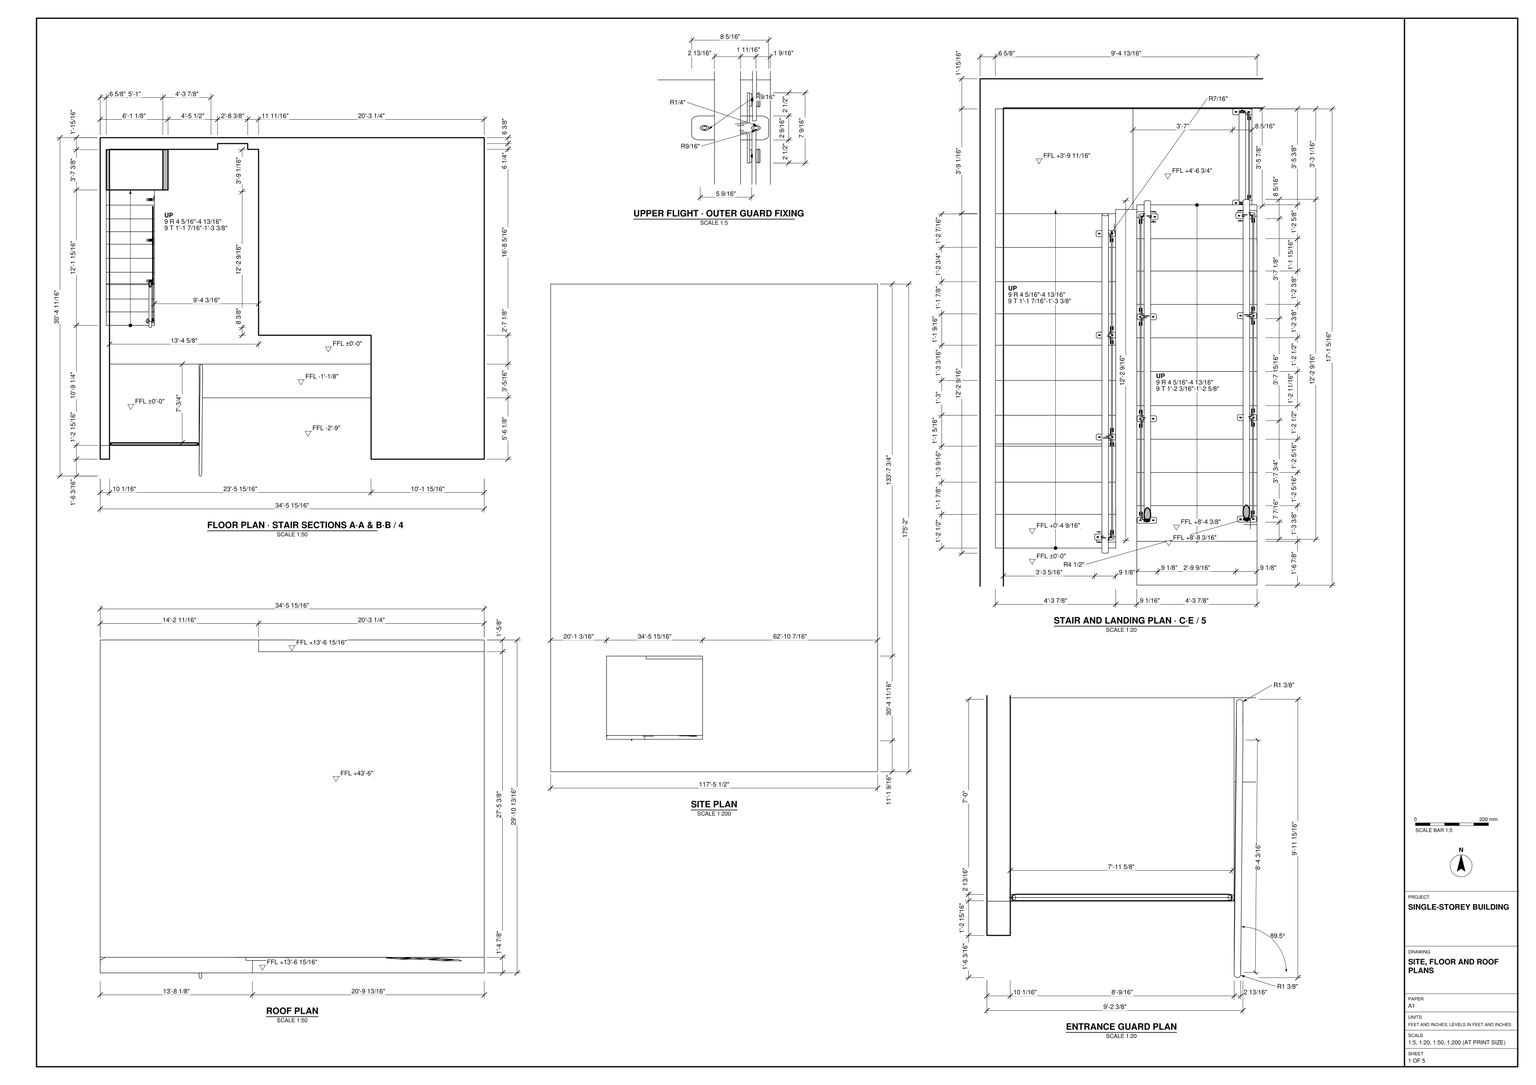
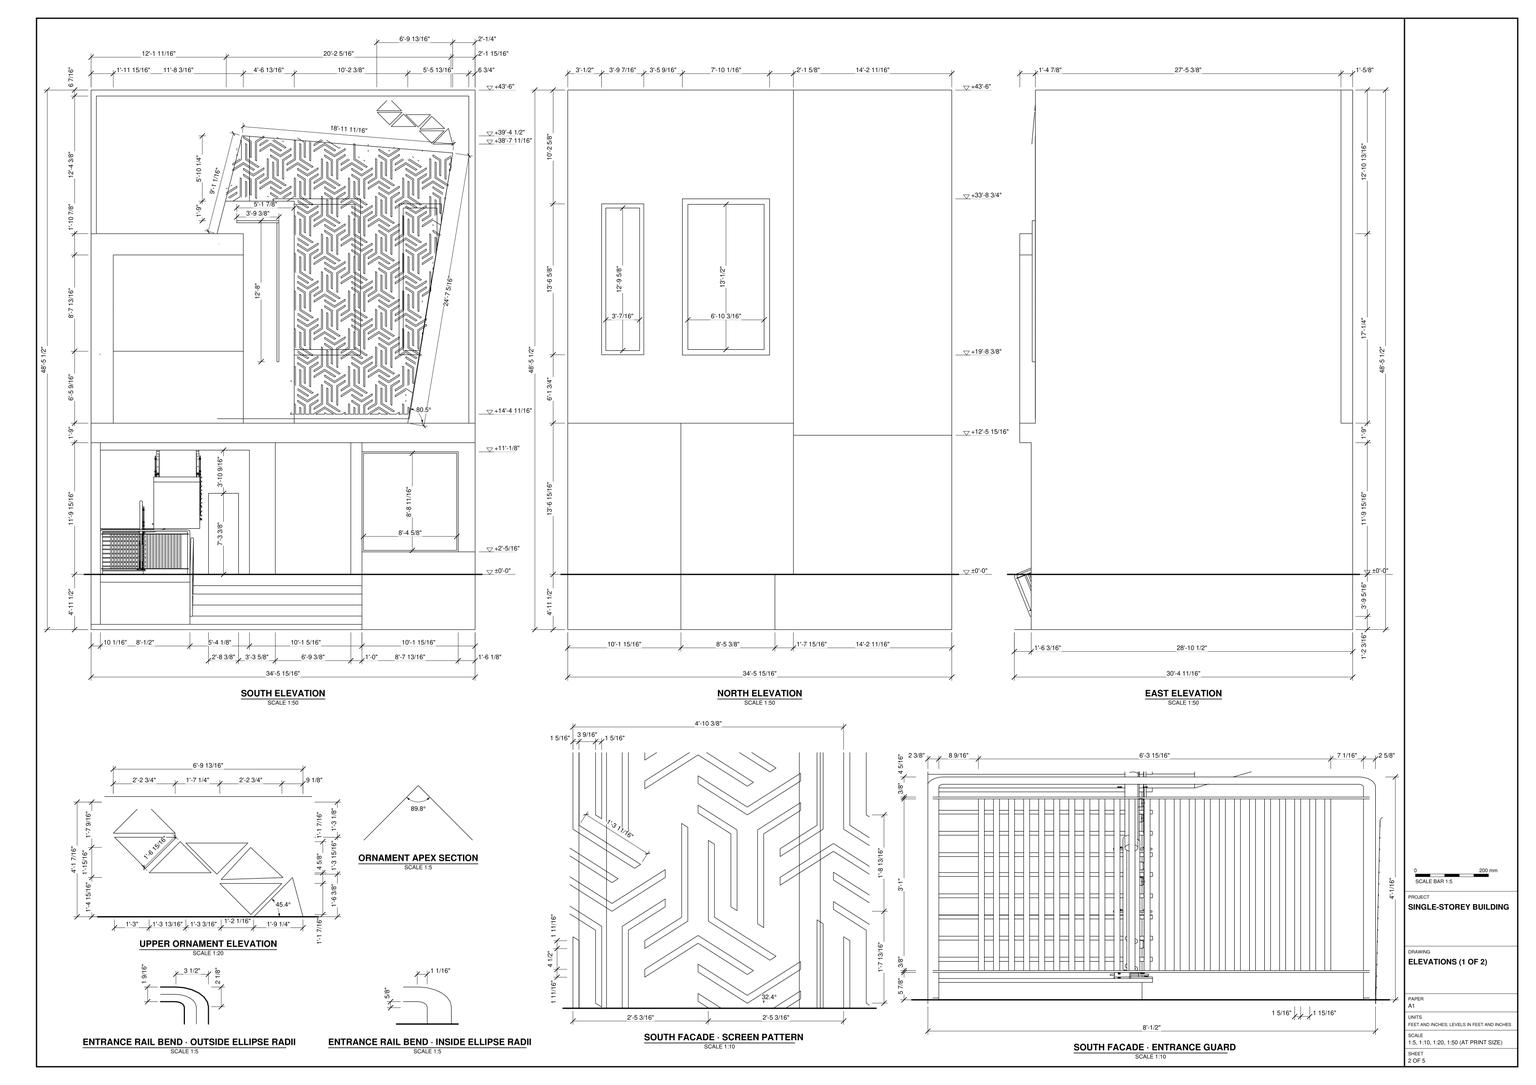
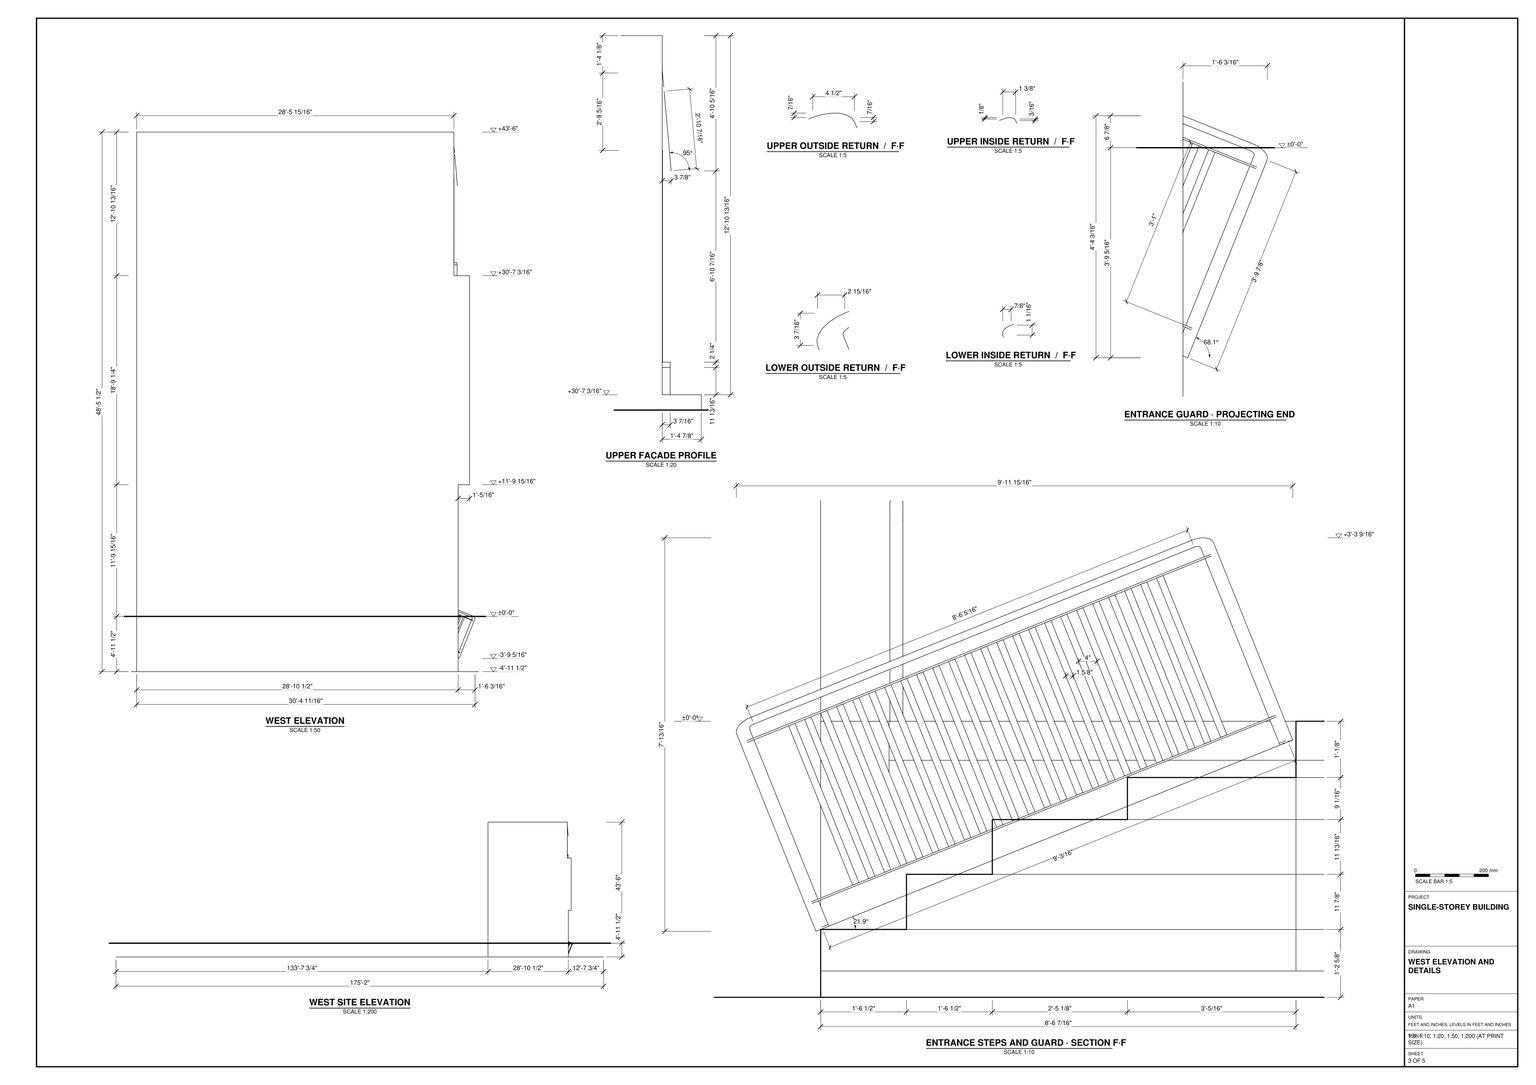
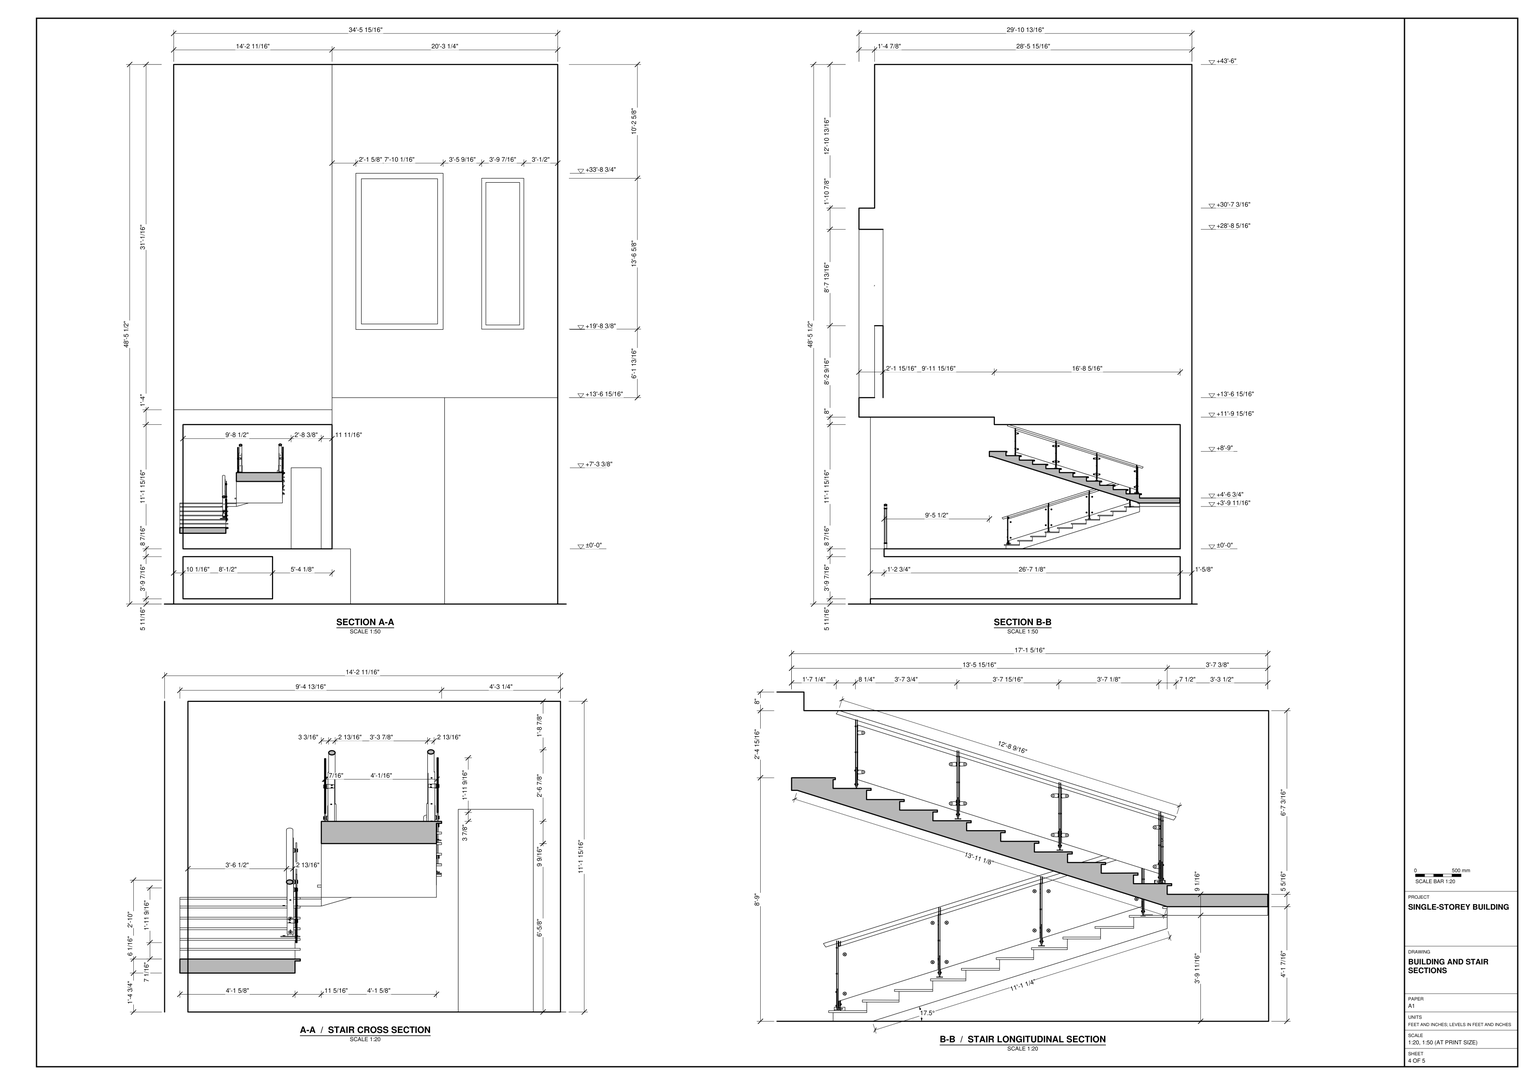
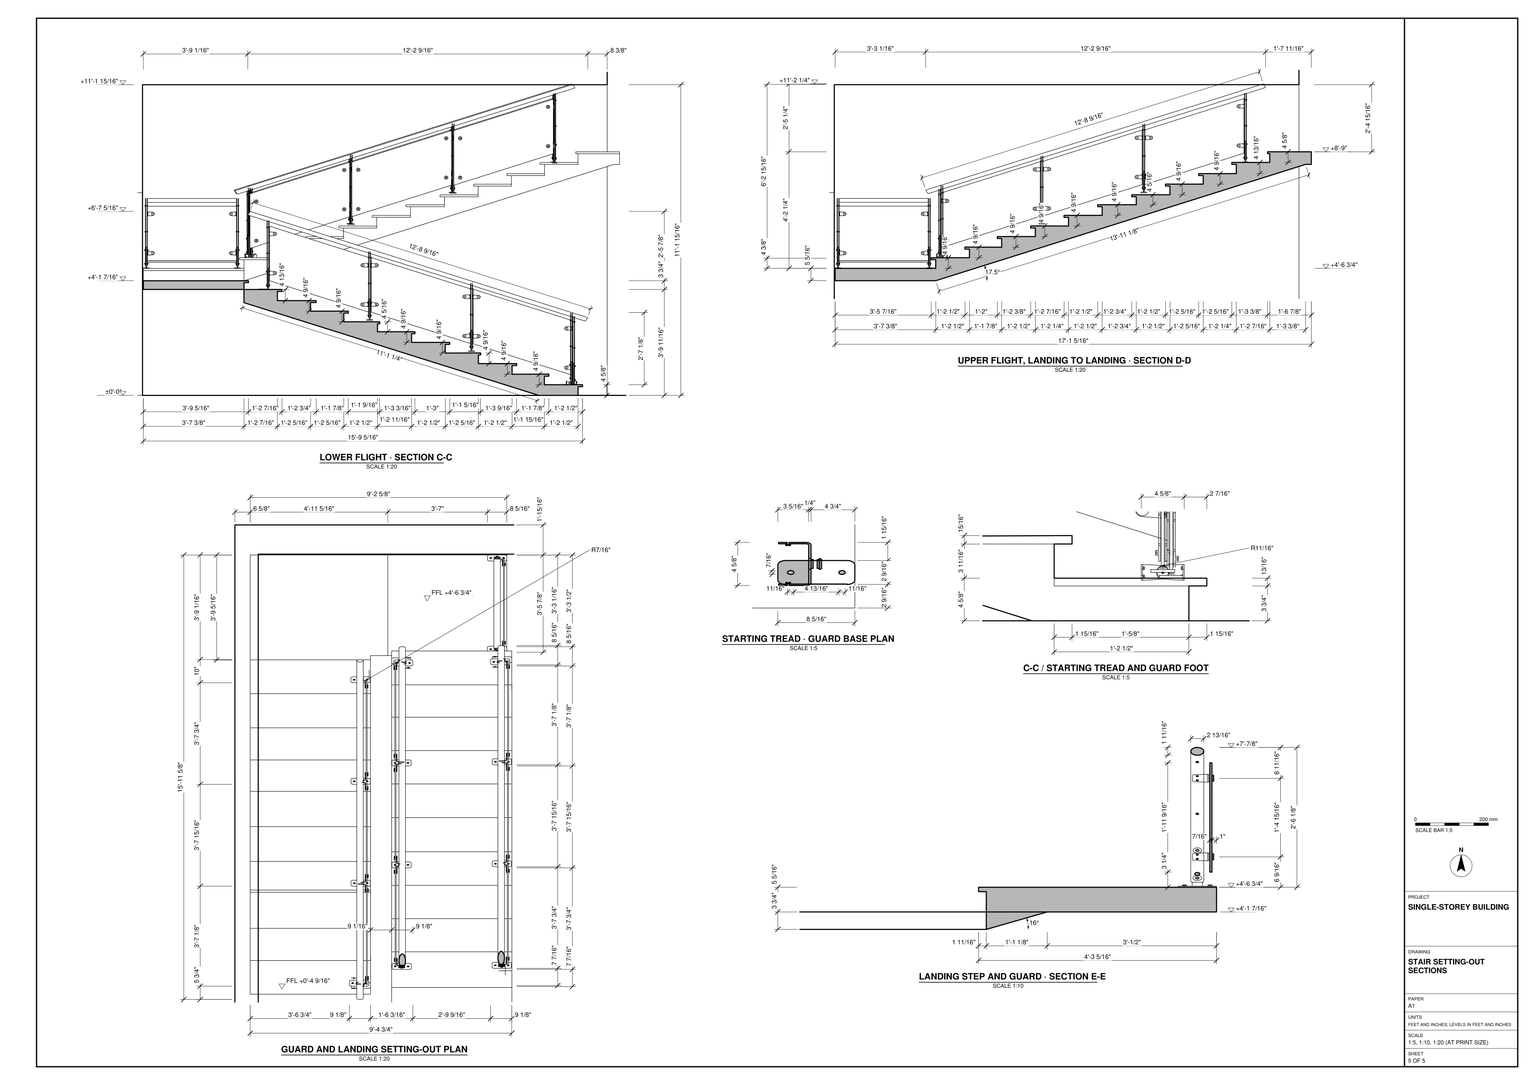
Work in feet and inches in SketchUp. Use task_files/diagram_01.pdf to model the building and its rectangular site. Including the site, the model measures 117'-5 1/2" along X, 175'-2" along Y and 48'-5 1/2" along Z. Use ±0'-0" as the ground-floor level. Position the building near the south end of the site, with more open ground to its east than to its west.

Build the walls, floor slabs and flat roof to the thicknesses and profiles shown. Use the elevations to place the framed openings and to set out the projections on the south facade. Model the sloping edges, notch and repeating angular pattern of the upper screen. Below it, form the entrance steps and landing, with the level guard across the landing and the sloping guard beside the steps. Follow the stair and landing plan for the two parallel flights; use the sections and fixing details to place the glass guards, posts and brackets along their edges.

Keep the walls, slabs and roof in separate groups or components. Group each furniture or joinery piece shown separately, and use components for repeated parts. Decor and loose items may be any suitable library components. Save one SketchUp model as output_files/single_storey_building_with_screened_facade_and_stairs.skp.

# SketchUp Ruby script. Lengths in inches.
U = 1.inch
M = Sketchup.active_model
def pt(a) = Geom::Point3d.new(a.map { |v| v * U })
def face(e, loops, mat)
  f = e.add_face(loops[0].map { |a| pt(a) })
  loops[1..].each { |l| e.add_face(l.map { |a| pt(a) }).erase! }
  f.material = f.back_material = mat if mat
  f
end
# faces: each face lists its corners as indices into pts; further lists are holes
def faces(e, pts, list, mat = nil) = list.each { |f| face(e, (f[0].is_a?(Array) ? f : [f]).map { |l| l.map { |i| pts[i] } }, mat) }
# xy, xz, yz: faces in a plane at the given z, y or x. An outline is a flat list of corners, or four numbers for a rectangle; further outlines are holes
def ring(l) = l.size == 4 ? [[l[0], l[1]], [l[2], l[1]], [l[2], l[3]], [l[0], l[3]]] : l.each_slice(2).to_a
def flat(e, list, mat, &to3) = list.each { |f| face(e, (f[0].is_a?(Array) ? f : [f]).map { |l| ring(l).map { |u, v| to3.(u, v) } }, mat) }
def xy(e, z, list, mat = nil) = flat(e, list, mat) { |x, y| [x, y, z] }
def xz(e, y, list, mat = nil) = flat(e, list, mat) { |x, z| [x, y, z] }
def yz(e, x, list, mat = nil) = flat(e, list, mat) { |y, z| [x, y, z] }
def lines(e, pts, list) = list.each { |a, b| e.add_line(pt(pts[a]), pt(pts[b])) }
# prism: a flat outline (further loops are holes) pulled along v
def prism(e, loops, v, mat = nil)
  f = face(e, loops, mat); d = Geom::Vector3d.new(v.map { |x| x * U })
  f.pushpull(f.normal.samedirection?(d) ? d.length : -d.length)
end
def box(e, o, s, mat = nil) = prism(e, [[o, [o[0] + s[0], o[1], o[2]], [o[0] + s[0], o[1] + s[1], o[2]], [o[0], o[1] + s[1], o[2]]]], [0, 0, s[2]], mat)
def at(x, y, z, deg = 0) = Geom::Transformation.translation(pt([x, y, z])) * Geom::Transformation.rotation(ORIGIN, Z_AXIS, deg.degrees)
def axes(o, x, y, z) = Geom::Transformation.new([*x, 0, *y, 0, *z, 0, *pt(o).to_a, 1])
def part(name) = M.definitions.add(name)
# library, detail: a bought-in or finely detailed component or shape, given as its bounding box
def library(name, o, s) = part(name).tap { |d| box(d.entities, o, s) }
def detail(e, o, s) = box(e.add_group.entities, o, s)
def put(e, d, t, mat = nil) = e.add_instance(d, t).tap { |i| i.material = mat if mat }
def group(e, t, mat = nil) = e.add_group.tap { |g| g.transformation = t; g.material = mat if mat }.entities
root = M.entities
M.materials.add("Niraj_Hair_Dark").color = [109, 109, 109]
M.materials.add("[0010_Snow]").color = [255, 250, 250]
M.materials.add("[Asphalt New]").color = [67, 60, 62]
M.materials.add("[Grass Dark Green]").color = [106, 157, 55]
M.materials.add("[Stone Coursed Rough]").color = [165, 160, 130]
M.materials.add("[Translucent Glass Gray]").color = [128, 128, 128]
M.materials["[Translucent Glass Gray]"].alpha = 0.5
M.materials.add("[Wood Floor Parquet]").color = [145, 89, 39]
M.materials.add("[Wood OSB]").color = [240, 195, 122]
c1 = library("Stairs\#2",[2342.14,0.12,0],[188.54,80.27,159.8125])
c2 = library("Group\#3",[1.59,0,0],[218.88,269.6875,1.18])
c3 = part("Patterned screen panel")
put(c3.entities,c2,at(3.9375,3.93,0))
c4 = part("CNC+PATTERN+DESIGN-1")
p = [[-487.64,162.15,197.43],[-460.46,162.15,303.05],[-233.53,162.15,284.47],[-280.48,162.01,-1.96],[-487.39,162.01,-1.96]]
lines(c4.entities,p,[[0,1],[1,2],[2,3],[3,4]])
put(c4.entities,c3,axes([-487.45,163.33,-1.96],[1.1232,0,0],[0,0,1.23552],[0,-1.1232,0]))
c5 = library("grille",[52.54,2.91,0],[58.66,1.57,48.03])
c6 = part("Group\#6")
xy(c6.entities,0,[[0,0,51.78,0,25.89,32]])
xy(root,0,[[241.17,151.76,655.09,498.26]])
xy(root,0,[[[0,0,1409.5,2102],[241.17,151.76,655.09,498.26]]],"[Grass Dark Green]")
xy(root,5.67,[[251.23,151.76,347.73,485.66]])
xy(root,14.625,[[347.73,151.76,533.15,170.26]])
xy(root,26.5,[[347.73,170.26,533.15,188.76]])
xy(root,38.3125,[[347.73,188.76,533.15,217.89]])
xy(root,47.375,[[347.73,217.89,533.15,254.22]])
xy(root,51.09,[[251.23,166.51,347.73,485.66]])
xy(root,59.5,[[241.17,151.76,251.23,166.51],[251.23,166.51,347.73,254.22],[251.23,254.22,533.15,254.22,533.15,285.32,411.85,285.32,411.85,485.66,400.14,485.66,400.14,491.91,367.76,491.91,367.76,485.66,251.23,485.66]])
xy(root,146.875,[[367.76,485.66,400.14,491.91]])
xy(root,193.42,[[251.23,285.32,411.85,485.66]])
xy(root,201.4375,[[241.17,139.45,251.23,151.76],[439.77,139.45,521.14,285.32],[533.15,139.45,655.09,151.76]])
xy(root,201.4375,[[251.23,139.45,439.77,285.32],[521.14,139.45,533.15,285.32]],"[Stone Coursed Rough]")
xy(root,222.4375,[[265.11,139.45,655.09,156.3],[411.85,485.66,655.09,498.26]])
xy(root,288.73,[[441.5,152.86,443.62,156.3]])
xy(root,300,[[265.11,156.3,405.29,165.41]])
xy(root,403.8125,[[265.11,139.45,405.29,165.41]],"[Wood Floor Parquet]")
xy(root,426.6875,[[241.17,139.45,405.29,139.45,405.29,156.3,246.91,156.3,241.17,153.1],[241.17,153.1,246.91,156.3,241.17,156.3]])
xy(root,438.48,[[398.25,152.86,441.5,156.3]])
xy(root,440.73,[[398.25,152.86,443.62,156.3]])
xy(root,581.5,[[241.17,156.3,655.09,156.3,655.09,485.66,411.85,485.66,411.85,498.26,241.17,498.26]])
xz(root,139.45,[[241.17,201.4375,655.09,222.4375],[241.17,222.4375,265.11,222.4375,265.11,403.8125,405.29,403.8125,405.29,426.6875,241.17,426.6875]],"[Asphalt New]")
xz(root,151.76,[[241.17,0,533.15,5.67],[241.17,5.67,251.23,59.5],[347.73,5.67,533.15,14.625],[241.17,59.5,251.23,201.4375],[[533.15,83.79,636.9375,191.62],[534.74,85.38,635.35,190.04]]])
xz(root,151.76,[[533.15,0,655.09,83.79],[636.9375,83.79,655.09,83.79,655.09,201.4375,533.15,201.4375,533.15,191.62,636.9375,191.62]],"[Stone Coursed Rough]")
xz(root,151.76,[[534.74,85.38,635.35,190.04]],"[Translucent Glass Gray]")
xz(root,152.86,[[441.5,288.73,443.62,438.48],[398.25,438.48,443.62,440.73]],"[Wood OSB]")
xz(root,156.3,[[582.47,222.4375,648.32,222.4375,648.32,575.05,246.91,575.05,246.91,426.6875,376.91,426.6875,385.9375,461.75,404.1,532.31,631.03,513.72]])
xz(root,156.3,[[[405.29,222.4375,460.1,222.4375,460.1,461.75,385.9375,461.75,376.91,426.6875,405.29,426.6875],[441.5,288.73,441.5,438.48,398.25,438.48,398.25,440.73,443.62,440.73,443.62,288.73]]],"Niraj_Hair_Dark")
xz(root,156.3,[[648.32,222.4375,655.09,222.4375,655.09,581.5,241.17,581.5,241.17,426.6875,246.91,426.6875,246.91,575.05,648.32,575.05]],"[0010_Snow]")
xz(root,165.41,[[265.11,222.4375,405.29,300]],"[Translucent Glass Gray]")
xz(root,166.51,[[251.23,51.09,347.73,59.5]])
xz(root,170.26,[[347.73,14.625,533.15,26.5]])
xz(root,188.76,[[347.73,26.5,533.15,38.3125]])
xz(root,217.89,[[347.73,38.3125,533.15,47.375]])
xz(root,254.22,[[347.73,47.375,533.15,59.5]])
xz(root,285.32,[[439.77,59.5,521.14,201.4375]])
xz(root,285.32,[[411.85,59.5,439.77,59.5,439.77,201.4375,251.23,201.4375,251.23,193.42,411.85,193.42],[521.14,59.5,533.15,201.4375]],"[Stone Coursed Rough]")
xz(root,485.66,[[251.23,5.67,347.73,51.09],[251.23,59.5,367.76,59.5,367.76,146.875,400.14,146.875,400.14,59.5,411.85,59.5,411.85,193.42,251.23,193.42],[[411.85,222.4375,655.09,581.5],[437.51,295.88,531.57,464.25],[573.14,296.23,618.57,458.86]]])
xz(root,485.66,[[[437.51,295.88,531.57,464.25],[443.46,301.83,525.62,458.3]],[[573.14,296.23,618.57,458.86],[577.64,300.74,614.07,454.36]]],"[Asphalt New]")
xz(root,485.66,[[577.64,300.74,614.07,454.36],[443.46,301.83,525.62,458.3]],"[Translucent Glass Gray]")
xz(root,491.91,[[367.76,59.5,400.14,146.875]],"[Wood Floor Parquet]")
xz(root,498.26,[[241.17,0,241.17,209.4375,411.85,209.4375,411.85,59.5,431.79,59.5,431.79,0],[431.79,0,431.79,59.5,411.85,59.5,411.85,222.4375,533.15,222.4375,533.15,0],[533.15,0,655.09,222.4375],[241.17,209.4375,411.85,581.5]])
yz(root,241.17,[[151.76,0,151.76,201.4375,139.45,201.4375,139.45,426.6875,156.3,426.6875,156.3,581.5,498.26,581.5,498.26,0]])
yz(root,251.23,[[151.76,5.67,485.66,5.67,485.66,51.09,166.51,51.09,166.51,59.5,151.76,59.5],[151.76,59.5,485.66,59.5,485.66,193.42,285.32,193.42,285.32,201.4375,151.76,201.4375]])
yz(root,265.11,[[139.45,222.4375,156.3,222.4375,156.3,300,165.41,300,165.41,403.8125,139.45,403.8125]])
yz(root,347.73,[[151.76,5.67,254.22,14.625],[254.22,5.67,485.66,14.625],[170.26,14.625,254.22,26.5],[254.22,14.625,485.66,26.5],[188.76,26.5,254.22,38.3125],
  [254.22,26.5,485.66,38.3125],[217.89,38.3125,254.22,47.375],[254.22,38.3125,485.66,47.375],[254.22,47.375,485.66,51.09],[166.51,51.09,254.22,59.5]])
yz(root,367.76,[[485.66,59.5,491.91,146.875]])
yz(root,398.25,[[152.86,438.48,156.3,440.73]])
yz(root,400.14,[[485.66,59.5,491.91,146.875]])
yz(root,405.29,[[156.3,300,165.41,403.8125],[139.45,403.8125,156.3,426.6875]])
yz(root,411.85,[[285.32,59.5,485.66,193.42],[485.66,222.4375,498.26,581.5]])
yz(root,441.5,[[152.86,288.73,156.3,438.48]])
yz(root,443.62,[[152.86,288.73,156.3,440.73]])
yz(root,533.15,[[151.76,14.625,151.76,81.81,266.7,81.81,266.7,191.62,151.76,191.62,151.76,201.4375,285.32,201.4375,285.32,59.5,254.22,59.5,254.22,47.375,217.89,47.375,217.89,38.3125,188.76,38.3125,188.76,26.5,170.26,26.5,170.26,14.625],[[151.76,81.81,266.7,191.62],[153.12,83.16,265.34,190.27]]])
yz(root,533.15,[[153.12,83.16,265.34,190.27]],"[Translucent Glass Gray]")
yz(root,655.09,[[151.76,0,498.26,0,498.26,222.4375,485.66,222.4375,485.66,581.5,156.3,581.5,156.3,222.4375,139.45,222.4375,139.45,201.4375,151.76,201.4375]])
p = [[347.73,166.51,48.59],[347.73,166.51,51.09],[250.54,139.45,296.33],[265.11,156.3,343.59],[379.25,139.45,415.75],[376.91,156.3,426.6875]]
lines(root,p,[[0,1],[2,3],[4,5]])
put(root,c1,axes([360.75,-2616.3,59.5],[0,1.2256,0],[-1.4054,0,0],[0,0,0.84]))
put(root,c4,at(864.55,-5.85,229.26))
put(root,c5,axes([164.35,174.67,59.5],[1.649,0,0],[0,-1.78,0],[0,0,1]))
put(root,c5,axes([357.62,345.51,92.44],[-0.01673,-1.75192,-0.70361],[-1.77993,0.01499,0.005],[-0.00053,-0.37268,0.92796]))
g1 = group(root,at(549.07,152.46,523.2))
put(g1,c6,axes([77.26,1.5,16.94],[-0.32269,-0.02889,-0.32724],[0.40278,-0.02315,-0.26217],[0,-0.99613,0.08795]),"[Asphalt New]")
put(g1,c6,axes([72.67,1.27,14.36],[-0.5161,0,0],[0,-0.03702,-0.41931],[0,-0.99613,0.08795]),"[Asphalt New]")
put(g1,c6,axes([0,3.18,36.02],[0.5161,0,0],[0,0.03702,0.41931],[0,-0.99613,0.08795]),"[Asphalt New]")
put(g1,c6,axes([27.25,3.03,34.29],[-0.5161,0,0],[0,-0.03702,-0.41931],[0,-0.99613,0.08795]),"[Asphalt New]")
put(g1,c6,axes([58.02,2.81,31.8],[-0.5161,0,0],[0,-0.03702,-0.41931],[0,-0.99613,0.08795]),"[Asphalt New]")
put(g1,c6,axes([15.5,1.68,18.98],[0.5161,0,0],[0,0.03702,0.41931],[0,-0.99613,0.08795]),"[Asphalt New]")
put(g1,c6,axes([46.5,1.42,16.0625],[0.51572,0.00142,0.0161],[-0.01981,0.03699,0.419],[0,-0.99613,0.08795]),"[Asphalt New]")
